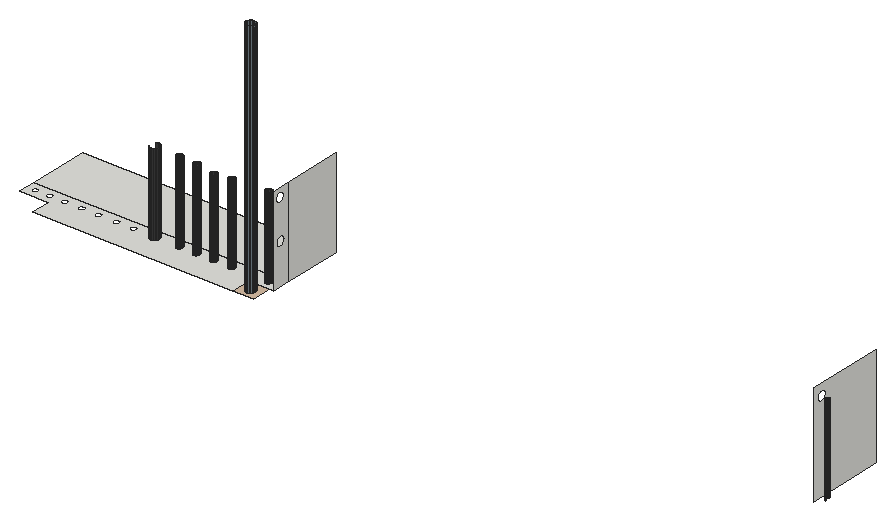
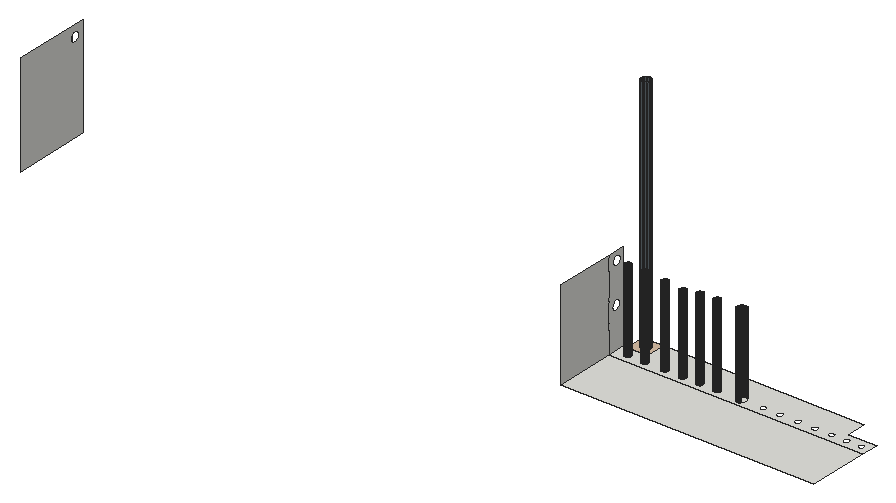
# SketchUp Ruby script. Lengths in inches.
U = 1.inch
M = Sketchup.active_model
def pt(a) = Geom::Point3d.new(a.map { |v| v * U })
def face(e, loops, mat)
  f = e.add_face(loops[0].map { |a| pt(a) })
  loops[1..].each { |l| e.add_face(l.map { |a| pt(a) }).erase! }
  f.material = f.back_material = mat if mat
  f
end
# faces: each face lists its corners as indices into pts; further lists are holes
def faces(e, pts, list, mat = nil) = list.each { |f| face(e, (f[0].is_a?(Array) ? f : [f]).map { |l| l.map { |i| pts[i] } }, mat) }
# xy, xz, yz: faces in a plane at the given z, y or x. An outline is a flat list of corners, or four numbers for a rectangle; further outlines are holes
def ring(l) = l.size == 4 ? [[l[0], l[1]], [l[2], l[1]], [l[2], l[3]], [l[0], l[3]]] : l.each_slice(2).to_a
def flat(e, list, mat, &to3) = list.each { |f| face(e, (f[0].is_a?(Array) ? f : [f]).map { |l| ring(l).map { |u, v| to3.(u, v) } }, mat) }
def xy(e, z, list, mat = nil) = flat(e, list, mat) { |x, y| [x, y, z] }
def xz(e, y, list, mat = nil) = flat(e, list, mat) { |x, z| [x, y, z] }
def yz(e, x, list, mat = nil) = flat(e, list, mat) { |y, z| [x, y, z] }
def lines(e, pts, list) = list.each { |a, b| e.add_line(pt(pts[a]), pt(pts[b])) }
# prism: a flat outline (further loops are holes) pulled along v
def prism(e, loops, v, mat = nil)
  f = face(e, loops, mat); d = Geom::Vector3d.new(v.map { |x| x * U })
  f.pushpull(f.normal.samedirection?(d) ? d.length : -d.length)
end
def box(e, o, s, mat = nil) = prism(e, [[o, [o[0] + s[0], o[1], o[2]], [o[0] + s[0], o[1] + s[1], o[2]], [o[0], o[1] + s[1], o[2]]]], [0, 0, s[2]], mat)
def at(x, y, z, deg = 0) = Geom::Transformation.translation(pt([x, y, z])) * Geom::Transformation.rotation(ORIGIN, Z_AXIS, deg.degrees)
def axes(o, x, y, z) = Geom::Transformation.new([*x, 0, *y, 0, *z, 0, *pt(o).to_a, 1])
def part(name) = M.definitions.add(name)
# library, detail: a bought-in or finely detailed component or shape, given as its bounding box
def library(name, o, s) = part(name).tap { |d| box(d.entities, o, s) }
def detail(e, o, s) = box(e.add_group.entities, o, s)
def put(e, d, t, mat = nil) = e.add_instance(d, t).tap { |i| i.material = mat if mat }
def group(e, t, mat = nil) = e.add_group.tap { |g| g.transformation = t; g.material = mat if mat }.entities
root = M.entities
M.materials.add("[Color M07]").color = [58, 58, 58]
M.materials.add("[Formica Laminate Dark]").color = [50, 53, 60]
M.materials.add("[Formica Laminate Light]").color = [213, 189, 164]
M.materials.add("[Formica Speckled Grey]").color = [112, 125, 132]
xy(root,479.18,[[[53.75,83.48,116.48,83.48,116.48,89.73,124.21,89.73,124.21,95.15,44.94,95.15,44.94,89.73,53.75,89.73],[84.85,90.875,84.44,90.93,84.0625,91.08,83.74,91.33,83.49,91.66,83.34,92.03,83.28,92.4375,83.34,92.84,83.49,93.22,83.74,93.54,84.0625,93.79,84.44,93.95,84.85,94,85.25,93.95,85.625,93.79,85.95,93.54,86.2,93.22,86.35,92.84,86.41,92.4375,86.35,92.03,86.2,91.66,85.95,91.33,85.625,91.08,85.25,90.93],[92.55,91.47,92.29,91.5,92.05,91.6,91.84,91.76,91.68,91.97,91.58,92.21,91.55,92.47,91.58,92.73,91.68,92.97,91.84,93.18,92.05,93.33,92.29,93.43,92.55,93.47,92.81,93.43,93.05,93.33,93.26,93.18,93.41,92.97,93.51,92.73,93.55,92.47,93.51,92.21,93.41,91.97,93.26,91.76,93.05,91.6,92.81,91.5],[120.49,91.47,120.23,91.5,119.99,91.6,119.78,91.76,119.62,91.97,119.52,92.21,119.49,92.47,119.52,92.73,119.62,92.97,119.78,93.18,119.99,93.33,120.23,93.43,120.49,93.47,120.74,93.43,120.99,93.33,121.19,93.18,121.35,92.97,121.45,92.73,121.49,92.47,121.45,92.21,121.35,91.97,121.19,91.76,120.99,91.6,120.74,91.5],[97.92,91.47,97.66,91.5,97.42,91.6,97.22,91.76,97.06,91.97,96.96,92.21,96.92,92.47,96.96,92.73,97.06,92.97,97.22,93.18,97.42,93.33,97.66,93.43,97.92,93.47,98.18,93.43,98.42,93.33,98.63,93.18,98.79,92.97,98.89,92.73,98.92,92.47,98.89,92.21,98.79,91.97,98.63,91.76,98.42,91.6,98.18,91.5],[115.11,91.47,114.85,91.5,114.61,91.6,114.4,91.76,114.24,91.97,114.14,92.21,114.11,92.47,114.14,92.73,114.24,92.97,114.4,93.18,114.61,93.33,114.85,93.43,115.11,93.47,115.37,93.43,115.61,93.33,115.82,93.18,115.98,92.97,116.08,92.73,116.11,92.47,116.08,92.21,115.98,91.97,115.82,91.76,115.61,91.6,115.37,91.5],[103.3,91.47,103.04,91.5,102.8,91.6,102.59,91.76,102.43,91.97,102.33,92.21,102.3,92.47,102.33,92.73,102.43,92.97,102.59,93.18,102.8,93.33,103.04,93.43,103.3,93.47,103.56,93.43,103.8,93.33,104.01,93.18,104.16,92.97,104.26,92.73,104.3,92.47,104.26,92.21,104.16,91.97,104.01,91.76,103.8,91.6,103.56,91.5],[108.86,91.47,108.6,91.5,108.36,91.6,108.15,91.76,107.99,91.97,107.89,92.21,107.86,92.47,107.89,92.73,107.99,92.97,108.15,93.18,108.36,93.33,108.6,93.43,108.86,93.47,109.12,93.43,109.36,93.33,109.57,93.18,109.73,92.97,109.83,92.73,109.86,92.47,109.83,92.21,109.73,91.97,109.57,91.76,109.36,91.6,109.12,91.5],[78.17,91.47,77.91,91.5,77.67,91.6,77.47,91.76,77.31,91.97,77.21,92.21,77.17,92.47,77.21,92.73,77.31,92.97,77.47,93.18,77.67,93.33,77.91,93.43,78.17,93.47,78.43,93.43,78.67,93.33,78.88,93.18,79.04,92.97,79.14,92.73,79.17,92.47,79.14,92.21,79.04,91.97,78.88,91.76,78.67,91.6,78.43,91.5],[52.05,91.47,51.79,91.5,51.55,91.6,51.34,91.76,51.18,91.97,51.08,92.21,51.05,92.47,51.08,92.73,51.18,92.97,51.34,93.18,51.55,93.33,51.79,93.43,52.05,93.47,52.31,93.43,52.55,93.33,52.76,93.18,52.91,92.97,53.01,92.73,53.05,92.47,53.01,92.21,52.91,91.97,52.76,91.76,52.55,91.6,52.31,91.5],[72.86,91.47,72.6,91.5,72.36,91.6,72.15,91.76,71.99,91.97,71.89,92.21,71.86,92.47,71.89,92.73,71.99,92.97,72.15,93.18,72.36,93.33,72.6,93.43,72.86,93.47,73.12,93.43,73.36,93.33,73.57,93.18,73.73,92.97,73.83,92.73,73.86,92.47,73.83,92.21,73.73,91.97,73.57,91.76,73.36,91.6,73.12,91.5],[56.74,91.47,56.48,91.5,56.24,91.6,56.03,91.76,55.87,91.97,55.77,92.21,55.74,92.47,55.77,92.73,55.87,92.97,56.03,93.18,56.24,93.33,56.48,93.43,56.74,93.47,56.99,93.43,57.24,93.33,57.44,93.18,57.6,92.97,57.7,92.73,57.74,92.47,57.7,92.21,57.6,91.97,57.44,91.76,57.24,91.6,56.99,91.5],[67.24,91.47,66.98,91.5,66.74,91.6,66.53,91.76,66.37,91.97,66.27,92.21,66.24,92.47,66.27,92.73,66.37,92.97,66.53,93.18,66.74,93.33,66.98,93.43,67.24,93.47,67.49,93.43,67.74,93.33,67.94,93.18,68.1,92.97,68.2,92.73,68.24,92.47,68.2,92.21,68.1,91.97,67.94,91.76,67.74,91.6,67.49,91.5],[61.92,91.47,61.66,91.5,61.42,91.6,61.22,91.76,61.06,91.97,60.96,92.21,60.92,92.47,60.96,92.73,61.06,92.97,61.22,93.18,61.42,93.33,61.66,93.43,61.92,93.47,62.18,93.43,62.42,93.33,62.63,93.18,62.79,92.97,62.89,92.73,62.92,92.47,62.89,92.21,62.79,91.97,62.63,91.76,62.42,91.6,62.18,91.5],[47.49,91.47,47.23,91.5,46.99,91.6,46.78,91.76,46.62,91.97,46.52,92.21,46.49,92.47,46.52,92.73,46.62,92.97,46.78,93.18,46.99,93.33,47.23,93.43,47.49,93.47,47.74,93.43,47.99,93.33,48.19,93.18,48.35,92.97,48.45,92.73,48.49,92.47,48.45,92.21,48.35,91.97,48.19,91.76,47.99,91.6,47.74,91.5]],[119.6875,84.95,119.3125,85,118.97,85.14,118.67,85.37,118.44,85.67,118.3,86.02,118.25,86.39,118.3,86.76,118.44,87.11,118.67,87.4,118.97,87.63,119.3125,87.78,119.6875,87.82,120.06,87.78,120.4,87.63,120.7,87.4,120.93,87.11,121.07,86.76,121.125,86.39,121.07,86.02,120.93,85.67,120.7,85.37,120.4,85.14,120.06,85],[84.85,90.875,84.44,90.93,84.0625,91.08,83.74,91.33,83.49,91.66,83.34,92.03,83.28,92.4375,83.34,92.84,83.49,93.22,83.74,93.54,84.0625,93.79,84.44,93.95,84.85,94,85.25,93.95,85.625,93.79,85.95,93.54,86.2,93.22,86.35,92.84,86.41,92.4375,86.35,92.03,86.2,91.66,85.95,91.33,85.625,91.08,85.25,90.93],[92.55,91.47,92.29,91.5,92.05,91.6,91.84,91.76,91.68,91.97,91.58,92.21,91.55,92.47,91.58,92.73,91.68,92.97,91.84,93.18,92.05,93.33,92.29,93.43,92.55,93.47,92.81,93.43,93.05,93.33,93.26,93.18,93.41,92.97,93.51,92.73,93.55,92.47,93.51,92.21,93.41,91.97,93.26,91.76,93.05,91.6,92.81,91.5],[97.92,91.47,97.66,91.5,97.42,91.6,97.22,91.76,97.06,91.97,96.96,92.21,96.92,92.47,96.96,92.73,97.06,92.97,97.22,93.18,97.42,93.33,97.66,93.43,97.92,93.47,98.18,93.43,98.42,93.33,98.63,93.18,98.79,92.97,98.89,92.73,98.92,92.47,98.89,92.21,98.79,91.97,98.63,91.76,98.42,91.6,98.18,91.5],
  [103.3,91.47,103.04,91.5,102.8,91.6,102.59,91.76,102.43,91.97,102.33,92.21,102.3,92.47,102.33,92.73,102.43,92.97,102.59,93.18,102.8,93.33,103.04,93.43,103.3,93.47,103.56,93.43,103.8,93.33,104.01,93.18,104.16,92.97,104.26,92.73,104.3,92.47,104.26,92.21,104.16,91.97,104.01,91.76,103.8,91.6,103.56,91.5],[108.86,91.47,108.6,91.5,108.36,91.6,108.15,91.76,107.99,91.97,107.89,92.21,107.86,92.47,107.89,92.73,107.99,92.97,108.15,93.18,108.36,93.33,108.6,93.43,108.86,93.47,109.12,93.43,109.36,93.33,109.57,93.18,109.73,92.97,109.83,92.73,109.86,92.47,109.83,92.21,109.73,91.97,109.57,91.76,109.36,91.6,109.12,91.5],[115.11,91.47,114.85,91.5,114.61,91.6,114.4,91.76,114.24,91.97,114.14,92.21,114.11,92.47,114.14,92.73,114.24,92.97,114.4,93.18,114.61,93.33,114.85,93.43,115.11,93.47,115.37,93.43,115.61,93.33,115.82,93.18,115.98,92.97,116.08,92.73,116.11,92.47,116.08,92.21,115.98,91.97,115.82,91.76,115.61,91.6,115.37,91.5],[120.49,91.47,120.23,91.5,119.99,91.6,119.78,91.76,119.62,91.97,119.52,92.21,119.49,92.47,119.52,92.73,119.62,92.97,119.78,93.18,119.99,93.33,120.23,93.43,120.49,93.47,120.74,93.43,120.99,93.33,121.19,93.18,121.35,92.97,121.45,92.73,121.49,92.47,121.45,92.21,121.35,91.97,121.19,91.76,120.99,91.6,120.74,91.5],[44.94,95.15,124.21,114.1]])
xy(root,479.18,[[[116.48,83.48,122.94,89.73],[119.6875,84.95,119.3125,85,118.97,85.14,118.67,85.37,118.44,85.67,118.3,86.02,118.25,86.39,118.3,86.76,118.44,87.11,118.67,87.4,118.97,87.63,119.3125,87.78,119.6875,87.82,120.06,87.78,120.4,87.63,120.7,87.4,120.93,87.11,121.07,86.76,121.125,86.39,121.07,86.02,120.93,85.67,120.7,85.37,120.4,85.14,120.06,85]]],"[Formica Laminate Light]")
yz(root,124.21,[[[89.73,479.18,95.15,506.99],[92.45,490.42,92.84,490.47,93.2,490.62,93.51,490.86,93.75,491.17,93.9,491.53,93.95,491.92,93.9,492.31,93.75,492.67,93.51,492.98,93.2,493.22,92.84,493.37,92.45,493.42,92.06,493.37,91.7,493.22,91.39,492.98,91.15,492.67,91,492.31,90.95,491.92,91,491.53,91.15,491.17,91.39,490.86,91.7,490.62,92.06,490.47],[92.15,502.86,92.52,502.91,92.87,503.05,93.16,503.28,93.39,503.58,93.53,503.92,93.58,504.3,93.53,504.67,93.39,505.01,93.16,505.3125,92.87,505.54,92.52,505.68,92.15,505.73,91.77,505.68,91.43,505.54,91.13,505.3125,90.9,505.01,90.76,504.67,90.71,504.3,90.76,503.92,90.9,503.58,91.13,503.28,91.43,503.05,91.77,502.91]],[95.15,479.18,114.1,506.99]])
yz(root,293.32,[[[89.73,479.47,114.1,511.22],[92.71,506.31,92.32,506.36,91.96,506.51,91.65,506.74,91.41,507.06,91.26,507.42,91.21,507.81,91.26,508.19,91.41,508.56,91.65,508.87,91.96,509.1,92.32,509.25,92.71,509.31,93.09,509.25,93.46,509.1,93.77,508.87,94.01,508.56,94.16,508.19,94.21,507.81,94.16,507.42,94.01,507.06,93.77,506.74,93.46,506.51,93.09,506.36]]])
p = [[119.3125,85,479.18],[119.6875,84.95,479.18],[119.6875,84.95,554.07],[119.3125,85,554.07],[120.06,85,479.18],[120.06,85,554.07],
  [118.97,85.14,479.18],[118.97,85.14,554.07],[120.4,85.14,479.18],[120.4,85.14,554.07],[118.67,85.37,479.18],[118.67,85.37,554.07],
  [120.7,85.37,479.18],[120.7,85.37,554.07],[118.44,85.67,479.18],[118.44,85.67,554.07],[120.93,85.67,479.18],[120.93,85.67,554.07],
  [118.3,86.02,479.18],[118.3,86.02,554.07],[121.07,86.02,479.18],[121.07,86.02,554.07],[118.25,86.39,479.18],[118.25,86.39,554.07],
  [121.125,86.39,479.18],[121.125,86.39,554.07],[118.3,86.76,479.18],[118.3,86.76,554.07],[121.07,86.76,479.18],[121.07,86.76,554.07],
  [118.44,87.11,479.18],[118.44,87.11,554.07],[120.93,87.11,479.18],[120.93,87.11,554.07],[118.67,87.4,479.18],[118.67,87.4,554.07],
  [120.7,87.4,479.18],[120.7,87.4,554.07],[118.97,87.63,479.18],[118.97,87.63,554.07],[120.4,87.63,479.18],[120.4,87.63,554.07],
  [119.3125,87.78,479.18],[119.3125,87.78,554.07],[120.06,87.78,479.18],[120.06,87.78,554.07],[119.6875,87.82,479.18],[119.6875,87.82,554.07],
  [84.0625,91.08,479.18],[84.44,90.93,479.18],[84.44,90.93,504.8],[84.0625,91.08,504.8],[84.85,90.875,479.18],[84.85,90.875,504.8],
  [85.25,90.93,479.18],[85.25,90.93,504.8],[85.625,91.08,479.18],[85.625,91.08,504.8],[83.74,91.33,479.18],[83.74,91.33,504.8],
  [85.95,91.33,479.18],[85.95,91.33,504.8],[86.2,91.66,479.18],[86.2,91.66,504.8],[92.05,91.6,479.18],[92.29,91.5,479.18],
  [92.29,91.5,504.67],[92.05,91.6,504.67],[92.55,91.47,479.18],[92.55,91.47,504.67],[92.81,91.5,479.18],[92.81,91.5,504.67],
  [93.05,91.6,479.18],[93.05,91.6,504.67],[97.42,91.6,479.18],[97.66,91.5,479.18],[97.66,91.5,504.43],[97.42,91.6,504.43],
  [97.92,91.47,479.18],[97.92,91.47,504.43],[98.18,91.5,479.18],[98.18,91.5,504.43],[98.42,91.6,479.18],[98.42,91.6,504.43],
  [102.8,91.6,479.18],[103.04,91.5,479.18],[103.04,91.5,503.49],[102.8,91.6,503.49],[103.3,91.47,479.18],[103.3,91.47,503.49],
  [103.56,91.5,479.18],[103.56,91.5,503.49],[103.8,91.6,479.18],[103.8,91.6,503.49],[108.36,91.6,479.18],[108.6,91.5,479.18],
  [108.6,91.5,504.05],[108.36,91.6,504.05],[108.86,91.47,479.18],[108.86,91.47,504.05],[109.12,91.5,479.18],[109.12,91.5,504.05],
  [109.36,91.6,479.18],[109.36,91.6,504.05],[114.61,91.6,479.18],[114.85,91.5,479.18],[114.85,91.5,504.67],[114.61,91.6,504.67],
  [115.11,91.47,479.18],[115.11,91.47,504.67],[115.37,91.5,479.18],[115.37,91.5,504.67],[115.61,91.6,479.18],[115.61,91.6,504.67],
  [119.99,91.6,479.18],[120.23,91.5,479.18],[120.23,91.5,504.67],[119.99,91.6,504.67],[120.49,91.47,479.18],[120.49,91.47,504.67],
  [120.74,91.5,479.18],[120.74,91.5,504.67],[120.99,91.6,479.18],[120.99,91.6,504.67],[91.84,91.76,479.18],[91.84,91.76,504.67],
  [93.26,91.76,479.18],[93.26,91.76,504.67],[97.22,91.76,479.18],[97.22,91.76,504.43],[98.63,91.76,479.18],[98.63,91.76,504.43],
  [102.59,91.76,479.18],[102.59,91.76,503.49],[104.01,91.76,479.18],[104.01,91.76,503.49],[108.15,91.76,479.18],[108.15,91.76,504.05],
  [109.57,91.76,479.18],[109.57,91.76,504.05],[114.4,91.76,479.18],[114.4,91.76,504.67],[115.82,91.76,479.18],[115.82,91.76,504.67],
  [119.78,91.76,479.18],[119.78,91.76,504.67],[121.19,91.76,479.18],[121.19,91.76,504.67],[86.35,92.03,479.18],[86.35,92.03,504.8],
  [91.68,91.97,479.18],[91.68,91.97,504.67],[93.41,91.97,479.18],[93.41,91.97,504.67],[97.06,91.97,479.18],[97.06,91.97,504.43],
  [98.79,91.97,479.18],[98.79,91.97,504.43],[102.43,91.97,479.18],[102.43,91.97,503.49],[104.16,91.97,479.18],[104.16,91.97,503.49],
  [107.99,91.97,479.18],[107.99,91.97,504.05],[109.73,91.97,479.18],[109.73,91.97,504.05],[114.24,91.97,479.18],[114.24,91.97,504.67],
  [115.98,91.97,479.18],[115.98,91.97,504.67],[119.62,91.97,479.18],[119.62,91.97,504.67],[121.35,91.97,479.18],[121.35,91.97,504.67],
  [86.41,92.4375,479.18],[86.41,92.4375,504.8],[91.58,92.21,479.18],[91.58,92.21,504.67],[93.51,92.21,479.18],[93.51,92.21,504.67],
  [96.96,92.21,479.18],[96.96,92.21,504.43],[98.89,92.21,479.18],[98.89,92.21,504.43],[102.33,92.21,479.18],[102.33,92.21,503.49],
  [104.26,92.21,479.18],[104.26,92.21,503.49],[107.89,92.21,479.18],[107.89,92.21,504.05],[109.83,92.21,479.18],[109.83,92.21,504.05],
  [114.14,92.21,479.18],[114.14,92.21,504.67],[116.08,92.21,479.18],[116.08,92.21,504.67],[119.52,92.21,479.18],[119.52,92.21,504.67],
  [121.45,92.21,479.18],[121.45,92.21,504.67],[91.55,92.47,479.18],[91.55,92.47,504.67],[93.55,92.47,479.18],[93.55,92.47,504.67],
  [96.92,92.47,479.18],[96.92,92.47,504.43],[98.92,92.47,479.18],[98.92,92.47,504.43],[102.3,92.47,479.18],[102.3,92.47,503.49],
  [104.3,92.47,479.18],[104.3,92.47,503.49],[107.86,92.47,479.18],[107.86,92.47,504.05],[109.86,92.47,479.18],[109.86,92.47,504.05],
  [114.11,92.47,479.18],[114.11,92.47,504.67],[116.11,92.47,479.18],[116.11,92.47,504.67],[119.49,92.47,479.18],[119.49,92.47,504.67],
  [121.49,92.47,479.18],[121.49,92.47,504.67],[86.35,92.84,479.18],[86.35,92.84,504.8],[91.58,92.73,479.18],[91.58,92.73,504.67],
  [93.51,92.73,479.18],[93.51,92.73,504.67],[96.96,92.73,479.18],[96.96,92.73,504.43],[98.89,92.73,479.18],[98.89,92.73,504.43],
  [102.33,92.73,479.18],[102.33,92.73,503.49],[104.26,92.73,479.18],[104.26,92.73,503.49],[107.89,92.73,479.18],[107.89,92.73,504.05],
  [109.83,92.73,479.18],[109.83,92.73,504.05],[114.14,92.73,479.18],[114.14,92.73,504.67],[116.08,92.73,479.18],[116.08,92.73,504.67],
  [119.52,92.73,479.18],[119.52,92.73,504.67],[121.45,92.73,479.18],[121.45,92.73,504.67],[91.68,92.97,479.18],[91.68,92.97,504.67],
  [93.41,92.97,479.18],[93.41,92.97,504.67],[97.06,92.97,479.18],[97.06,92.97,504.43],[98.79,92.97,479.18],[98.79,92.97,504.43],
  [102.43,92.97,479.18],[102.43,92.97,503.49],[104.16,92.97,479.18],[104.16,92.97,503.49],[107.99,92.97,479.18],[107.99,92.97,504.05],
  [109.73,92.97,479.18],[109.73,92.97,504.05],[114.24,92.97,479.18],[114.24,92.97,504.67],[115.98,92.97,479.18],[115.98,92.97,504.67],
  [119.62,92.97,479.18],[119.62,92.97,504.67],[121.35,92.97,479.18],[121.35,92.97,504.67],[86.2,93.22,479.18],[86.2,93.22,504.8],
  [91.84,93.18,479.18],[91.84,93.18,504.67],[93.26,93.18,479.18],[93.26,93.18,504.67],[97.22,93.18,479.18],[97.22,93.18,504.43],
  [98.63,93.18,479.18],[98.63,93.18,504.43],[102.59,93.18,479.18],[102.59,93.18,503.49],[104.01,93.18,479.18],[104.01,93.18,503.49],
  [108.15,93.18,479.18],[108.15,93.18,504.05],[109.57,93.18,479.18],[109.57,93.18,504.05],[114.4,93.18,479.18],[114.4,93.18,504.67],
  [115.82,93.18,479.18],[115.82,93.18,504.67],[119.78,93.18,479.18],[119.78,93.18,504.67],[121.19,93.18,479.18],[121.19,93.18,504.67],
  [85.95,93.54,479.18],[85.95,93.54,504.8],[92.05,93.33,479.18],[92.05,93.33,504.67],[93.05,93.33,479.18],[93.05,93.33,504.67],
  [97.42,93.33,479.18],[97.42,93.33,504.43],[98.42,93.33,479.18],[98.42,93.33,504.43],[102.8,93.33,479.18],[102.8,93.33,503.49],
  [103.8,93.33,479.18],[103.8,93.33,503.49],[108.36,93.33,479.18],[108.36,93.33,504.05],[109.36,93.33,479.18],[109.36,93.33,504.05],
  [114.61,93.33,479.18],[114.61,93.33,504.67],[115.61,93.33,479.18],[115.61,93.33,504.67],[119.99,93.33,479.18],[119.99,93.33,504.67],
  [120.99,93.33,479.18],[120.99,93.33,504.67],[92.29,93.43,479.18],[92.29,93.43,504.67],[92.81,93.43,479.18],[92.81,93.43,504.67],
  [97.66,93.43,479.18],[97.66,93.43,504.43],[98.18,93.43,479.18],[98.18,93.43,504.43],[103.04,93.43,479.18],[103.04,93.43,503.49],
  [103.56,93.43,479.18],[103.56,93.43,503.49],[108.6,93.43,479.18],[108.6,93.43,504.05],[109.12,93.43,479.18],[109.12,93.43,504.05],
  [114.85,93.43,479.18],[114.85,93.43,504.67],[115.37,93.43,479.18],[115.37,93.43,504.67],[120.23,93.43,479.18],[120.23,93.43,504.67],
  [120.74,93.43,479.18],[120.74,93.43,504.67],[92.55,93.47,479.18],[92.55,93.47,504.67],[97.92,93.47,479.18],[97.92,93.47,504.43],
  [103.3,93.47,479.18],[103.3,93.47,503.49],[108.86,93.47,479.18],[108.86,93.47,504.05],[115.11,93.47,479.18],[115.11,93.47,504.67],
  [120.49,93.47,479.18],[120.49,93.47,504.67],[85.625,93.79,479.18],[85.625,93.79,504.8],[84.44,93.95,479.18],[84.0625,93.79,479.18],
  [84.0625,93.79,504.8],[84.44,93.95,504.8],[84.44,93.95,491.92],[85.25,93.95,479.18],[85.25,93.95,491.92],[85.25,93.95,504.8],
  [84.85,94,479.18],[84.85,94,504.8],[294.97,92.02,479.47],[295.18,91.93,479.47],[295.18,91.93,507.47],[294.97,92.02,507.47],
  [295.4,91.9,479.47],[295.4,91.9,507.47],[294.78,92.16,479.47],[294.78,92.16,507.47],[294.65,92.34,479.47],[294.65,92.34,507.47],
  [294.56,92.55,479.47],[294.56,92.55,507.47],[294.53,92.78,479.47],[294.53,92.78,507.47],[294.56,93.01,479.47],[294.56,93.01,507.47],
  [294.65,93.22,479.47],[294.65,93.22,507.47],[294.78,93.4,479.47],[294.78,93.4,507.47],[294.97,93.54,479.47],[294.97,93.54,507.47],
  [295.18,93.625,479.47],[295.18,93.625,507.47]]
faces(root,p,[[0,1,2,3],[1,4,5,2],[6,0,3,7],[4,8,9,5],[10,6,7,11],[8,12,13,9],[14,10,11,15],[12,16,17,13],
  [18,14,15,19],[16,20,21,17],[22,18,19,23],[20,24,25,21],[26,22,23,27],[24,28,29,25],[30,26,27,31],[28,32,33,29],
  [34,30,31,35],[32,36,37,33],[38,34,35,39],[36,40,41,37],[42,38,39,43],[40,44,45,41],[46,42,43,47],[44,46,47,45]],"[Formica Speckled Grey]")
faces(root,p,[[48,49,50,51],[49,52,53,50],[52,54,55,53],[54,56,57,55],[58,48,51,59],[56,60,61,57],[60,62,63,61],[64,65,66,67],
  [65,68,69,66],[68,70,71,69],[70,72,73,71],[74,75,76,77],[75,78,79,76],[78,80,81,79],[80,82,83,81],[84,85,86,87],
  [85,88,89,86],[88,90,91,89],[90,92,93,91],[94,95,96,97],[95,98,99,96],[98,100,101,99],[100,102,103,101],[104,105,106,107],
  [105,108,109,106],[108,110,111,109],[110,112,113,111],[114,115,116,117],[115,118,119,116],[118,120,121,119],[120,122,123,121],[124,64,67,125],
  [72,126,127,73],[128,74,77,129],[82,130,131,83],[132,84,87,133],[92,134,135,93],[136,94,97,137],[102,138,139,103],[140,104,107,141],
  [112,142,143,113],[144,114,117,145],[122,146,147,123],[62,148,149,63],[150,124,125,151],[126,152,153,127],[154,128,129,155],[130,156,157,131],
  [158,132,133,159],[134,160,161,135],[162,136,137,163],[138,164,165,139],[166,140,141,167],[142,168,169,143],[170,144,145,171],[146,172,173,147],
  [148,174,175,149],[176,150,151,177],[152,178,179,153],[180,154,155,181],[156,182,183,157],[184,158,159,185],[160,186,187,161],[188,162,163,189],
  [164,190,191,165],[192,166,167,193],[168,194,195,169],[196,170,171,197],[172,198,199,173],[200,176,177,201],[178,202,203,179],[204,180,181,205],
  [182,206,207,183],[208,184,185,209],[186,210,211,187],[212,188,189,213],[190,214,215,191],[216,192,193,217],[194,218,219,195],[220,196,197,221],
  [198,222,223,199],[174,224,225,175],[226,200,201,227],[202,228,229,203],[230,204,205,231],[206,232,233,207],[234,208,209,235],[210,236,237,211],
  [238,212,213,239],[214,240,241,215],[242,216,217,243],[218,244,245,219],[246,220,221,247],[222,248,249,223],[250,226,227,251],[228,252,253,229],
  [254,230,231,255],[232,256,257,233],[258,234,235,259],[236,260,261,237],[262,238,239,263],[240,264,265,241],[266,242,243,267],[244,268,269,245],
  [270,246,247,271],[248,272,273,249],[224,274,275,225],[276,250,251,277],[252,278,279,253],[280,254,255,281],[256,282,283,257],[284,258,259,285],
  [260,286,287,261],[288,262,263,289],[264,290,291,265],[292,266,267,293],[268,294,295,269],[296,270,271,297],[272,298,299,273],[274,300,301,275],
  [302,276,277,303],[278,304,305,279],[306,280,281,307],[282,308,309,283],[310,284,285,311],[286,312,313,287],[314,288,289,315],[290,316,317,291],
  [318,292,293,319],[294,320,321,295],[322,296,297,323],[298,324,325,299],[326,302,303,327],[304,328,329,305],[330,306,307,331],[308,332,333,309],
  [334,310,311,335],[312,336,337,313],[338,314,315,339],[316,340,341,317],[342,318,319,343],[320,344,345,321],[346,322,323,347],[324,348,349,325],
  [350,326,327,351],[328,350,351,329],[352,330,331,353],[332,352,353,333],[354,334,335,355],[336,354,355,337],[356,338,339,357],[340,356,357,341],
  [358,342,343,359],[344,358,359,345],[360,346,347,361],[348,360,361,349],[300,362,363,301],[364,365,366,367,368],[362,369,370,371,363],[372,364,368,367,373],
  [369,372,373,371,370]],"[Color M07]")
faces(root,p,[[374,375,376,377],[375,378,379,376],[380,374,377,381],[382,380,381,383],[384,382,383,385],[386,384,385,387],[388,386,387,389],[390,388,389,391],
  [392,390,391,393],[394,392,393,395],[396,394,395,397]],"[Formica Laminate Dark]")
